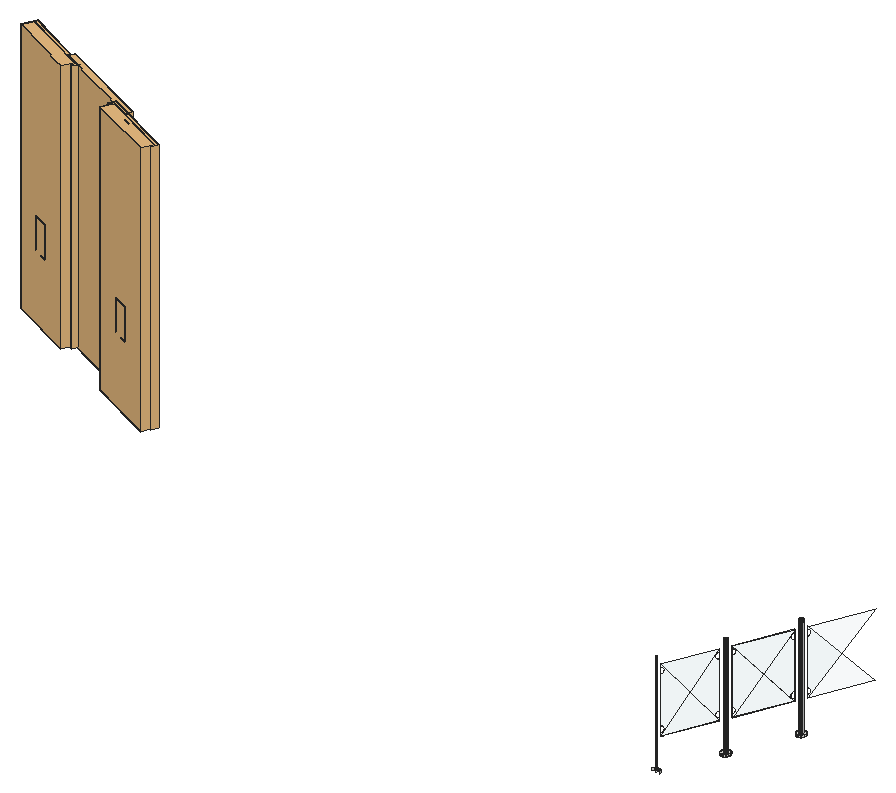
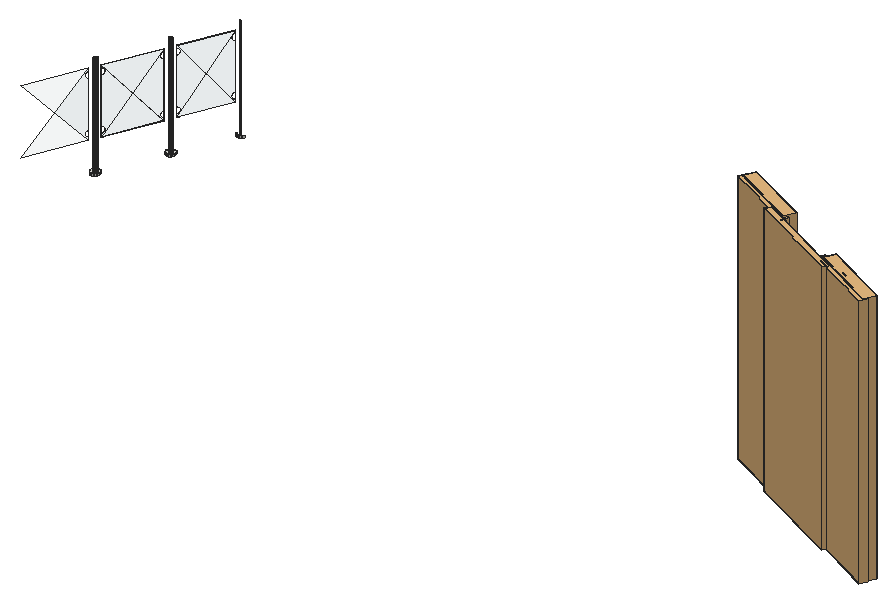
# SketchUp Ruby script. Lengths in inches.
U = 1.inch
M = Sketchup.active_model
def pt(a) = Geom::Point3d.new(a.map { |v| v * U })
def face(e, loops, mat)
  f = e.add_face(loops[0].map { |a| pt(a) })
  loops[1..].each { |l| e.add_face(l.map { |a| pt(a) }).erase! }
  f.material = f.back_material = mat if mat
  f
end
# faces: each face lists its corners as indices into pts; further lists are holes
def faces(e, pts, list, mat = nil) = list.each { |f| face(e, (f[0].is_a?(Array) ? f : [f]).map { |l| l.map { |i| pts[i] } }, mat) }
# xy, xz, yz: faces in a plane at the given z, y or x. An outline is a flat list of corners, or four numbers for a rectangle; further outlines are holes
def ring(l) = l.size == 4 ? [[l[0], l[1]], [l[2], l[1]], [l[2], l[3]], [l[0], l[3]]] : l.each_slice(2).to_a
def flat(e, list, mat, &to3) = list.each { |f| face(e, (f[0].is_a?(Array) ? f : [f]).map { |l| ring(l).map { |u, v| to3.(u, v) } }, mat) }
def xy(e, z, list, mat = nil) = flat(e, list, mat) { |x, y| [x, y, z] }
def xz(e, y, list, mat = nil) = flat(e, list, mat) { |x, z| [x, y, z] }
def yz(e, x, list, mat = nil) = flat(e, list, mat) { |y, z| [x, y, z] }
def lines(e, pts, list) = list.each { |a, b| e.add_line(pt(pts[a]), pt(pts[b])) }
# prism: a flat outline (further loops are holes) pulled along v
def prism(e, loops, v, mat = nil)
  f = face(e, loops, mat); d = Geom::Vector3d.new(v.map { |x| x * U })
  f.pushpull(f.normal.samedirection?(d) ? d.length : -d.length)
end
def box(e, o, s, mat = nil) = prism(e, [[o, [o[0] + s[0], o[1], o[2]], [o[0] + s[0], o[1] + s[1], o[2]], [o[0], o[1] + s[1], o[2]]]], [0, 0, s[2]], mat)
def at(x, y, z, deg = 0) = Geom::Transformation.translation(pt([x, y, z])) * Geom::Transformation.rotation(ORIGIN, Z_AXIS, deg.degrees)
def axes(o, x, y, z) = Geom::Transformation.new([*x, 0, *y, 0, *z, 0, *pt(o).to_a, 1])
def part(name) = M.definitions.add(name)
# library, detail: a bought-in or finely detailed component or shape, given as its bounding box
def library(name, o, s) = part(name).tap { |d| box(d.entities, o, s) }
def detail(e, o, s) = box(e.add_group.entities, o, s)
def put(e, d, t, mat = nil) = e.add_instance(d, t).tap { |i| i.material = mat if mat }
def group(e, t, mat = nil) = e.add_group.tap { |g| g.transformation = t; g.material = mat if mat }.entities
root = M.entities
M.materials.add("Glass_Safety_01").color = [204, 235, 244]
M.materials["Glass_Safety_01"].alpha = 0.1
M.materials.add("[Color_000]").color = [255, 255, 255]
c1 = library("Group14",[-64.97,9.24,0.31],[138.52,9.93,292.57])
c2 = library("Group16",[86.37,-10.76,76.46],[21.79,14.87,35.97])
c3 = library("Group22",[48.82,-10.91,0.23],[97.72,18.57,293.12])
c4 = library("Group24",[44.03,2.01,0.26],[103.73,11,292.35])
c5 = library("Group27",[-106.21,-10.76,76.46],[21.8,14.87,35.97])
c6 = library("Group35",[-145.81,2.01,0.26],[103.73,11,292.35])
c7 = library("Group33",[-144.59,-10.91,0.23],[97.72,18.57,293.12])
c8 = part("Group\#71")
put(c8.entities,c1,at(145.81,10.91,-0.23))
put(c8.entities,c2,at(145.81,10.91,-0.23))
put(c8.entities,c3,at(145.81,10.91,-0.23))
put(c8.entities,c4,at(145.81,10.91,-0.23))
put(c8.entities,c5,at(145.81,10.91,-0.23))
put(c8.entities,c6,at(145.81,10.91,-0.23))
put(c8.entities,c7,at(145.81,10.91,-0.23))
xy(root,321.27,[[[916.89,703.23,917.3,703.3125,917.66,703.5,917.97,703.77,918.2,704.11,918.33,704.5,918.35,704.91,918.27,705.32,918.09,705.68,917.8125,705.99,917.47,706.22,917.08,706.35,916.67,706.37,916.27,706.29,915.9,706.11,915.59,705.83,915.37,705.49,915.24,705.1,915.21,704.6875,915.29,704.29,915.48,703.92,915.75,703.61,916.09,703.39,916.16,703.36,916.48,703.26],[916.83,704.17,916.66,704.18,916.53,704.23,916.51,704.24,916.37,704.33,916.26,704.45,916.1875,704.6,916.15,704.76,916.16,704.92,916.22,705.08,916.31,705.21,916.43,705.32,916.58,705.4,916.74,705.43,916.9,705.42,917.03,705.375,917.06,705.37,917.19,705.28,917.3,705.16,917.38,705.01,917.41,704.85,917.4,704.68,917.35,704.53,917.26,704.39,917.14,704.28,916.99,704.21]],[916.16,703.36,916.53,704.23,916.51,704.24,916.37,704.33,916.26,704.45,916.1875,704.6,916.15,704.76,916.16,704.92,916.22,705.08,916.31,705.21,916.43,705.32,916.58,705.4,916.74,705.43,916.9,705.42,917.03,705.375,917.41,706.24,917.08,706.35,916.67,706.37,916.27,706.29,915.9,706.11,915.59,705.83,915.37,705.49,915.24,705.1,915.21,704.6875,915.29,704.29,915.48,703.92,915.75,703.61,916.09,703.39],[916.53,704.23,917.03,705.375,916.9,705.42,916.74,705.43,916.58,705.4,916.43,705.32,916.31,705.21,916.22,705.08,916.16,704.92,916.15,704.76,916.1875,704.6,916.26,704.45,916.37,704.33,916.51,704.24],[[926.125,724.43,926.53,724.51,926.9,724.69,927.2,724.97,927.43,725.31,927.56,725.7,927.58,726.11,927.5,726.51,927.32,726.88,927.04,727.1875,926.7,727.41,926.64,727.43,926.3125,727.54,925.9,727.57,925.5,727.49,925.13,727.3,924.82,727.03,924.6,726.6875,924.47,726.3,924.44,725.89,924.53,725.48,924.71,725.11,924.98,724.81,925.33,724.58,925.72,724.45],[926.06,725.37,925.89,725.38,925.76,725.42,925.74,725.43,925.6,725.52,925.49,725.64,925.42,725.79,925.39,725.95,925.39,726.12,925.45,726.27,925.54,726.41,925.66,726.52,925.81,726.59,925.97,726.625,926.13,726.62,926.26,726.57,926.29,726.5625,926.43,726.47,926.53,726.35,926.61,726.2,926.64,726.04,926.63,725.88,926.58,725.72,926.49,725.59,926.37,725.48,926.22,725.4]],[925.39,724.56,925.76,725.42,925.74,725.43,925.6,725.52,925.49,725.64,925.42,725.79,925.39,725.95,925.39,726.12,925.45,726.27,925.54,726.41,925.66,726.52,925.81,726.59,925.97,726.625,926.13,726.62,926.26,726.57,926.64,727.43,926.3125,727.54,925.9,727.57,925.5,727.49,925.13,727.3,924.82,727.03,924.6,726.6875,924.47,726.3,924.44,725.89,924.53,725.48,924.71,725.11,924.98,724.81,925.33,724.58],
  [925.76,725.42,926.26,726.57,926.13,726.62,925.97,726.625,925.81,726.59,925.66,726.52,925.54,726.41,925.45,726.27,925.39,726.12,925.39,725.95,925.42,725.79,925.49,725.64,925.6,725.52,925.74,725.43]])
xy(root,321.27,[[916.83,704.17,916.99,704.21,917.14,704.28,917.26,704.39,917.35,704.53,917.4,704.68,917.41,704.85,917.38,705.01,917.3,705.16,917.19,705.28,917.06,705.37,917.03,705.375,916.53,704.23,916.66,704.18],[926.06,725.37,926.22,725.4,926.37,725.48,926.49,725.59,926.58,725.72,926.63,725.88,926.64,726.04,926.61,726.2,926.53,726.35,926.43,726.47,926.29,726.5625,926.26,726.57,925.76,725.42,925.89,725.38]],"[Color_000]")
xy(root,321.86,[[916.89,703.23,917.3,703.3125,917.66,703.5,917.97,703.77,918.2,704.11,918.33,704.5,918.35,704.91,918.27,705.32,918.09,705.68,917.8125,705.99,917.47,706.22,917.08,706.35,916.67,706.37,916.27,706.29,915.9,706.11,915.59,705.83,915.37,705.49,915.24,705.1,915.21,704.6875,915.29,704.29,915.48,703.92,915.75,703.61,916.09,703.39,916.48,703.26],[926.125,724.43,926.53,724.51,926.9,724.69,927.2,724.97,927.43,725.31,927.56,725.7,927.58,726.11,927.5,726.51,927.32,726.88,927.04,727.1875,926.7,727.41,926.3125,727.54,925.9,727.57,925.5,727.49,925.13,727.3,924.82,727.03,924.6,726.6875,924.47,726.3,924.44,725.89,924.53,725.48,924.71,725.11,924.98,724.81,925.33,724.58,925.72,724.45]])
xy(root,331.9,[[908.9375,686.55,908.76,686.625,916.16,703.12],[908.76,686.625,915.98,703.2,916.16,703.12],[917.66,706.57,917.48,706.65,925.38,724.31],[917.48,706.65,925.2,724.39,925.38,724.31]],"Glass_Safety_01")
yz(root,925.39,[[725.95,321.27,726.12,357.27]],"[Color_000]")
p = [[908.34,685.35,321.27],[908.3125,685.36,321.27],[908.18,685.4,321.27],[908.18,685.4,357.27],[908.34,685.35,357.27],[909.55,685.3,321.27],
  [909.37,685.66,321.27],[909.37,685.66,321.86],[909.55,685.3,321.86],[908.02,685.41,321.27],[907.86,685.375,321.27],[907.86,685.375,357.27],
  [908.02,685.41,357.27],[906.87,685.8125,321.27],[906.65,685.47,321.27],[906.65,685.47,321.86],[906.87,685.8125,321.86],[909.09,685.97,321.27],
  [909.09,685.97,321.86],[907.18,686.09,321.27],[907.18,686.09,321.86],[908.75,686.2,321.27],[908.75,686.2,321.86],[907.55,686.27,321.27],
  [907.55,686.27,321.86],[908.6875,686.22,321.27],[908.36,686.33,321.27],[908.36,686.33,321.86],[907.95,686.35,321.27],[907.95,686.35,321.86],
  [916.48,703.26,321.27],[916.89,703.23,321.27],[916.89,703.23,321.86],[916.48,703.26,321.86],[917.3,703.3125,321.27],[917.3,703.3125,321.86],
  [916.09,703.39,321.27],[916.16,703.36,321.27],[916.09,703.39,321.86],[917.66,703.5,321.27],[917.66,703.5,321.86],[915.75,703.61,321.27],
  [915.75,703.61,321.86],[917.97,703.77,321.27],[917.97,703.77,321.86],[915.48,703.92,321.27],[915.48,703.92,321.86],[918.2,704.11,321.27],
  [918.2,704.11,321.86],[915.29,704.29,321.27],[915.29,704.29,321.86],[918.33,704.5,321.27],[918.33,704.5,321.86],[916.37,704.33,321.27],
  [916.51,704.24,321.27],[916.51,704.24,357.27],[916.37,704.33,357.27],[916.53,704.23,321.27],[916.66,704.18,321.27],[916.66,704.18,357.27],
  [916.83,704.17,321.27],[916.83,704.17,357.27],[916.99,704.21,321.27],[916.99,704.21,357.27],[917.14,704.28,321.27],[917.14,704.28,357.27],
  [915.21,704.6875,321.27],[915.21,704.6875,321.86],[916.26,704.45,321.27],[916.26,704.45,357.27],[917.26,704.39,321.27],[917.26,704.39,357.27],
  [916.1875,704.6,321.27],[916.1875,704.6,357.27],[917.35,704.53,321.27],[917.35,704.53,357.27],[917.4,704.68,321.27],[917.4,704.68,357.27],
  [918.35,704.91,321.27],[918.35,704.91,321.86],[916.15,704.76,321.27],[916.15,704.76,357.27],[915.24,705.1,321.27],[915.24,705.1,321.86],
  [917.41,704.85,321.27],[917.41,704.85,357.27],[916.16,704.92,321.27],[916.16,704.92,357.27],[917.38,705.01,321.27],[917.38,705.01,357.27],
  [916.22,705.08,321.27],[916.22,705.08,357.27],[918.27,705.32,321.27],[918.27,705.32,321.86],[917.3,705.16,321.27],[917.3,705.16,357.27],
  [915.37,705.49,321.27],[915.37,705.49,321.86],[916.31,705.21,321.27],[916.31,705.21,357.27],[916.43,705.32,321.27],[916.43,705.32,357.27],
  [917.19,705.28,321.27],[917.19,705.28,357.27],[916.58,705.4,321.27],[916.58,705.4,357.27],[917.06,705.37,321.27],[917.06,705.37,357.27],
  [918.09,705.68,321.27],[918.09,705.68,321.86],[916.74,705.43,321.27],[916.74,705.43,357.27],[916.9,705.42,321.27],[916.9,705.42,357.27],
  [917.03,705.375,321.27],[915.59,705.83,321.27],[915.59,705.83,321.86],[917.8125,705.99,321.27],[917.8125,705.99,321.86],[915.9,706.11,321.27],
  [915.9,706.11,321.86],[917.47,706.22,321.27],[917.47,706.22,321.86],[916.27,706.29,321.27],[916.27,706.29,321.86],[917.41,706.24,321.27],
  [917.08,706.35,321.27],[917.08,706.35,321.86],[916.67,706.37,321.27],[916.67,706.37,321.86],[925.72,724.45,321.27],[926.125,724.43,321.27],
  [926.125,724.43,321.86],[925.72,724.45,321.86],[926.53,724.51,321.27],[926.53,724.51,321.86],[925.33,724.58,321.27],[925.39,724.56,321.27],
  [925.33,724.58,321.86],[926.9,724.69,321.27],[926.9,724.69,321.86],[924.98,724.81,321.27],[924.98,724.81,321.86],[927.2,724.97,321.27],
  [927.2,724.97,321.86],[924.71,725.11,321.27],[924.71,725.11,321.86],[927.43,725.31,321.27],[927.43,725.31,321.86],[924.53,725.48,321.27],
  [924.53,725.48,321.86],[925.6,725.52,321.27],[925.74,725.43,321.27],[925.74,725.43,357.27],[925.6,725.52,357.27],[925.76,725.42,321.27],
  [925.89,725.38,321.27],[925.89,725.38,357.27],[926.06,725.37,321.27],[926.06,725.37,357.27],[926.22,725.4,321.27],[926.22,725.4,357.27],
  [926.37,725.48,321.27],[926.37,725.48,357.27],[924.44,725.89,321.27],[924.44,725.89,321.86],[925.49,725.64,321.27],[925.49,725.64,357.27],
  [926.49,725.59,321.27],[926.49,725.59,357.27],[925.42,725.79,321.27],[925.42,725.79,357.27],[926.58,725.72,321.27],[926.58,725.72,357.27],
  [926.63,725.88,321.27],[926.63,725.88,357.27],[925.39,725.95,321.27],[925.39,725.95,357.27],[924.47,726.3,321.27],[924.47,726.3,321.86],
  [926.64,726.04,321.27],[926.64,726.04,357.27],[926.61,726.2,321.27],[926.61,726.2,357.27],[925.45,726.27,321.27],[925.39,726.12,321.27],
  [925.39,726.12,357.27],[925.45,726.27,357.27],[926.53,726.35,321.27],[926.53,726.35,357.27],[924.6,726.6875,321.27],[924.6,726.6875,321.86],
  [925.54,726.41,321.27],[925.54,726.41,357.27],[925.66,726.52,321.27],[925.66,726.52,357.27],[926.43,726.47,321.27],[926.43,726.47,357.27],
  [925.81,726.59,321.27],[925.81,726.59,357.27],[926.29,726.5625,321.27],[926.29,726.5625,357.27],[927.5,726.51,321.27],[927.32,726.88,321.27],
  [927.32,726.88,321.86],[927.5,726.51,321.86],[925.97,726.625,321.27],[925.97,726.625,357.27],[926.13,726.62,321.27],[926.13,726.62,357.27],
  [926.26,726.57,321.27],[924.82,727.03,321.27],[924.82,727.03,321.86],[927.04,727.1875,321.27],[927.04,727.1875,321.86],[925.13,727.3,321.27],
  [925.13,727.3,321.86],[926.7,727.41,321.27],[926.7,727.41,321.86],[925.5,727.49,321.27],[925.5,727.49,321.86],[926.64,727.43,321.27],
  [926.3125,727.54,321.27],[926.3125,727.54,321.86],[925.9,727.57,321.27],[925.9,727.57,321.86],[908.76,686.625,331.9],[908.9375,686.55,331.9],
  [908.9375,686.55,333],[908.9375,686.55,335.125],[908.9375,686.55,351.28],[908.9375,686.55,353.41],[908.9375,686.55,354.51],[908.76,686.625,354.51],
  [908.76,686.625,353.41],[908.76,686.625,351.28],[908.76,686.625,335.125],[908.76,686.625,333],[909.05,686.8,335.09],[909.15,687.03,334.98],
  [909.24,687.24,334.8125],[909.31,687.39,334.59],[909.35,687.49,334.34],[909.36,687.52,334.0625],[909.35,687.49,333.79],[909.31,687.39,333.53],
  [909.24,687.24,333.3125],[909.15,687.03,333.14],[909.05,686.8,333.04],[916.16,703.12,354.51],[909.05,686.8,353.37],[909.15,687.03,353.27],
  [909.24,687.24,353.1],[909.31,687.39,352.88],[909.35,687.49,352.62],[909.36,687.52,352.35],[909.35,687.49,352.07],[909.31,687.39,351.8125],
  [909.24,687.24,351.59],[909.15,687.03,351.43],[909.05,686.8,351.32],[916.16,703.12,331.9],[916.16,703.12,333],[916.09,702.96,333],
  [915.98,702.71,333.04],[915.875,702.47,333.14],[915.79,702.27,333.3125],[915.72,702.11,333.53],[915.68,702.02,333.79],[915.66,701.98,334.0625],
  [915.68,702.02,334.34],[915.72,702.11,334.59],[915.79,702.27,334.8125],[915.875,702.47,334.98],[915.98,702.71,335.09],[916.09,702.96,335.125],
  [916.16,703.12,335.125],[916.16,703.12,351.28],[916.09,702.96,351.28],[915.98,702.71,351.32],[915.875,702.47,351.43],[915.79,702.27,351.59],
  [915.72,702.11,351.8125],[915.68,702.02,352.07],[915.66,701.98,352.35],[915.68,702.02,352.62],[915.72,702.11,352.88],[915.79,702.27,353.1],
  [915.875,702.47,353.27],[915.98,702.71,353.37],[916.09,702.96,353.41],[916.16,703.12,353.41],[908.87,686.88,333.04],[908.97,687.11,333.14],
  [909.06,687.3125,333.3125],[909.125,687.47,333.53],[909.17,687.57,333.79],[909.18,687.6,334.0625],[909.17,687.57,334.34],[909.125,687.47,334.59],
  [909.06,687.3125,334.8125],[908.97,687.11,334.98],[908.87,686.88,335.09],[908.87,686.88,351.32],[908.97,687.11,351.43],[909.06,687.3125,351.59],
  [909.125,687.47,351.8125],[909.17,687.57,352.07],[909.18,687.6,352.35],[909.17,687.57,352.62],[909.125,687.47,352.88],[909.06,687.3125,353.1],
  [908.97,687.11,353.27],[908.87,686.88,353.37],[915.98,703.2,331.9],[915.98,703.2,351.28],[915.98,703.2,335.125],[915.91,703.04,335.125],
  [915.8,702.78,335.09],[915.69,702.55,334.98],[915.61,702.35,334.8125],[915.54,702.19,334.59],[915.5,702.1,334.34],[915.48,702.0625,334.0625],
  [915.5,702.1,333.79],[915.54,702.19,333.53],[915.61,702.35,333.3125],[915.69,702.55,333.14],[915.8,702.78,333.04],[915.91,703.04,333],
  [915.98,703.2,333],[915.98,703.2,354.51],[915.98,703.2,353.41],[915.91,703.04,353.41],[915.8,702.78,353.37],[915.69,702.55,353.27],
  [915.61,702.35,353.1],[915.54,702.19,352.88],[915.5,702.1,352.62],[915.48,702.0625,352.35],[915.5,702.1,352.07],[915.54,702.19,351.8125],
  [915.61,702.35,351.59],[915.69,702.55,351.43],[915.8,702.78,351.32],[915.91,703.04,351.28],[917.48,706.65,331.9],[917.66,706.57,331.9],
  [917.66,706.57,333],[917.66,706.57,335.125],[917.66,706.57,351.28],[917.66,706.57,353.41],[917.66,706.57,354.51],[917.48,706.65,354.51],
  [917.48,706.65,353.41],[917.48,706.65,351.28],[917.48,706.65,335.125],[917.48,706.65,333],[917.59,706.9,333.04],[917.69,707.13,333.14],
  [917.78,707.34,333.3125],[917.85,707.49,333.53],[917.89,707.59,333.79],[917.9,707.62,334.0625],[917.89,707.59,334.34],[917.85,707.49,334.59],
  [917.78,707.34,334.8125],[917.69,707.13,334.98],[917.59,706.9,335.09],[917.59,706.9,351.32],[917.69,707.13,351.43],[917.78,707.34,351.59],
  [917.85,707.49,351.8125],[917.89,707.59,352.07],[917.9,707.62,352.35],[917.89,707.59,352.62],[917.85,707.49,352.88],[917.78,707.34,353.1],
  [917.69,707.13,353.27],[917.59,706.9,353.37],[925.2,724.39,331.9],[925.2,724.39,351.28],[925.2,724.39,335.125],[925.14,724.23,335.125],
  [925.03,723.98,335.09],[924.92,723.74,334.98],[924.84,723.54,334.8125],[924.77,723.39,334.59],[924.73,723.29,334.34],[924.71,723.26,334.0625],
  [924.73,723.29,333.79],[924.77,723.39,333.53],[924.84,723.54,333.3125],[924.92,723.74,333.14],[925.03,723.98,333.04],[925.14,724.23,333],
  [925.2,724.39,333],[925.2,724.39,354.51],[925.2,724.39,353.41],[925.14,724.23,353.41],[925.03,723.98,353.37],[924.92,723.74,353.27],
  [924.84,723.54,353.1],[924.77,723.39,352.88],[924.73,723.29,352.62],[924.71,723.26,352.35],[924.73,723.29,352.07],[924.77,723.39,351.8125],
  [924.84,723.54,351.59],[924.92,723.74,351.43],[925.03,723.98,351.32],[925.14,724.23,351.28],[917.77,706.82,335.09],[917.87,707.05,334.98],
  [917.96,707.26,334.8125],[918.03,707.41,334.59],[918.07,707.51,334.34],[918.08,707.54,334.0625],[918.07,707.51,333.79],[918.03,707.41,333.53],
  [917.96,707.26,333.3125],[917.87,707.05,333.14],[917.77,706.82,333.04],[925.38,724.31,354.51],[917.77,706.82,353.37],[917.87,707.05,353.27],
  [917.96,707.26,353.1],[918.03,707.41,352.88],[918.07,707.51,352.62],[918.08,707.54,352.35],[918.07,707.51,352.07],[918.03,707.41,351.8125],
  [917.96,707.26,351.59],[917.87,707.05,351.43],[917.77,706.82,351.32],[925.38,724.31,331.9],[925.38,724.31,333],[925.32,724.15,333],
  [925.21,723.9,333.04],[925.11,723.67,333.14],[925.02,723.46,333.3125],[924.95,723.31,333.53],[924.91,723.21,333.79],[924.89,723.18,334.0625],
  [924.91,723.21,334.34],[924.95,723.31,334.59],[925.02,723.46,334.8125],[925.11,723.67,334.98],[925.21,723.9,335.09],[925.32,724.15,335.125],
  [925.38,724.31,335.125],[925.38,724.31,351.28],[925.32,724.15,351.28],[925.21,723.9,351.32],[925.11,723.67,351.43],[925.02,723.46,351.59],
  [924.95,723.31,351.8125],[924.91,723.21,352.07],[924.89,723.18,352.35],[924.91,723.21,352.62],[924.95,723.31,352.88],[925.02,723.46,353.1],
  [925.11,723.67,353.27],[925.21,723.9,353.37],[925.32,724.15,353.41],[925.38,724.31,353.41],[926.71,727.84,331.9],[926.89,727.76,331.9],
  [926.89,727.76,333],[926.89,727.76,335.125],[926.89,727.76,351.28],[926.89,727.76,353.41],[926.89,727.76,354.51],[926.71,727.84,354.51],
  [926.71,727.84,353.41],[926.71,727.84,351.28],[926.71,727.84,335.125],[926.71,727.84,333],[926.82,728.09,333.04],[926.92,728.33,333.14],
  [927.01,728.53,333.3125],[927.08,728.6875,333.53],[927.12,728.78,333.79],[927.13,728.82,334.0625],[927.12,728.78,334.34],[927.08,728.6875,334.59],
  [927.01,728.53,334.8125],[926.92,728.33,334.98],[926.82,728.09,335.09],[926.82,728.09,351.32],[926.92,728.33,351.43],[927.01,728.53,351.59],
  [927.08,728.6875,351.8125],[927.12,728.78,352.07],[927.13,728.82,352.35],[927.12,728.78,352.62],[927.08,728.6875,352.88],[927.01,728.53,353.1],
  [926.92,728.33,353.27],[926.82,728.09,353.37],[935.125,747.16,331.9],[927,728.02,335.09],[927.1,728.25,334.98],[927.19,728.45,334.8125],
  [927.26,728.61,334.59],[927.3,728.7,334.34],[927.3125,728.74,334.0625],[927.3,728.7,333.79],[927.26,728.61,333.53],[927.19,728.45,333.3125],
  [927.1,728.25,333.14],[927,728.02,333.04],[935.3,747.08,354.51],[927,728.02,353.37],[927.1,728.25,353.27],[927.19,728.45,353.1],
  [927.26,728.61,352.88],[927.3,728.7,352.62],[927.3125,728.74,352.35],[927.3,728.7,352.07],[927.26,728.61,351.8125],[927.19,728.45,351.59],
  [927.1,728.25,351.43],[927,728.02,351.32]]
faces(root,p,[[0,1,2,3,4],[9,10,11,12],[2,9,12,3],[53,54,55,56],[54,57,58,59,55],[58,60,61,59],[60,62,63,61],[62,64,65,63],
  [68,53,56,69],[64,70,71,65],[72,68,69,73],[70,74,75,71],[74,76,77,75],[80,72,73,81],[76,84,85,77],[86,80,81,87],
  [84,88,89,85],[90,86,87,91],[88,94,95,89],[98,90,91,99],[100,98,99,101],[94,102,103,95],[104,100,101,105],[102,106,107,103],
  [110,104,105,111],[112,110,111,113],[106,114,112,113,107],[151,152,153,154],[152,155,156,157,153],[156,158,159,157],[158,160,161,159],[160,162,163,161],
  [166,151,154,167],[162,168,169,163],[170,166,167,171],[168,172,173,169],[172,174,175,173],[176,170,171,177],[174,180,181,175],[180,182,183,181],
  [184,185,186,187],[182,188,189,183],[192,184,187,193],[194,192,193,195],[188,196,197,189],[198,194,195,199],[196,200,201,197],[206,198,199,207],
  [208,206,207,209],[200,210,208,209,201]],"[Color_000]")
faces(root,p,[[5,6,7,8],[13,14,15,16],[6,17,18,7],[19,13,16,20],[17,21,22,18],[23,19,20,24],[21,25,26,27,22],[28,23,24,29],
  [26,28,29,27],[30,31,32,33],[31,34,35,32],[36,37,30,33,38],[34,39,40,35],[41,36,38,42],[39,43,44,40],[45,41,42,46],
  [43,47,48,44],[49,45,46,50],[47,51,52,48],[66,49,50,67],[51,78,79,52],[82,66,67,83],[78,92,93,79],[96,82,83,97],
  [92,108,109,93],[115,96,97,116],[108,117,118,109],[119,115,116,120],[117,121,122,118],[123,119,120,124],[121,125,126,127,122],[128,123,124,129],
  [126,128,129,127],[130,131,132,133],[131,134,135,132],[136,137,130,133,138],[134,139,140,135],[141,136,138,142],[139,143,144,140],[145,141,142,146],
  [143,147,148,144],[149,145,146,150],[164,149,150,165],[178,164,165,179],[190,178,179,191],[202,203,204,205],[211,190,191,212],[203,213,214,204],
  [215,211,212,216],[213,217,218,214],[219,215,216,220],[217,221,222,223,218],[224,219,220,225],[222,224,225,223]])
faces(root,p,[[226,227,228,229,230,231,232,233,234,235,236,237],[230,229,238,239,240,241,242,243,244,245,246,247,248,228,227,249,232,231,250,251,252,253,254,255,256,257,258,259,260],[261,262,263,264,265,266,267,268,269,270,271,272,273,274,275,276,277,278,279,280,281,282,283,284,285,286,287,288,289,290,291,249,227],[226,237,292,293,294,295,296,297,298,299,300,301,302,236,235,303,304,305,306,307,308,309,310,311,312,313,234,233,314],[315,316,317,318,319,320,321,322,323,324,325,326,327,328,329,330,314,233,331,332,333,334,335,336,337,338,339,340,341,342,343,344,345],[261,314,330,316,315,332,331,249,291,277,276,262],[346,347,348,349,350,351,352,353,354,355,356,357],[346,357,358,359,360,361,362,363,364,365,366,367,368,356,355,369,370,371,372,373,374,375,376,377,378,379,354,353,380],
  [381,382,383,384,385,386,387,388,389,390,391,392,393,394,395,396,380,353,397,398,399,400,401,402,403,404,405,406,407,408,409,410,411],[350,349,412,413,414,415,416,417,418,419,420,421,422,348,347,423,352,351,424,425,426,427,428,429,430,431,432,433,434],[435,436,437,438,439,440,441,442,443,444,445,446,447,448,449,450,451,452,453,454,455,456,457,458,459,460,461,462,463,464,465,423,347],[435,380,396,382,381,398,397,423,465,451,450,436],[466,467,468,469,470,471,472,473,474,475,476,477],[466,477,478,479,480,481,482,483,484,485,486,487,488,476,475,489,490,491,492,493,494,495,496,497,498,499,474,473,500],[470,469,501,502,503,504,505,506,507,508,509,510,511,468,467,512,472,471,513,514,515,516,517,518,519,520,521,522,523]],"Glass_Safety_01")
put(root,c8,axes([616.02,773.82,324.57],[0.23478,-0.11401,0],[0.09657,0.19887,0],[0,0,0.30131]))
